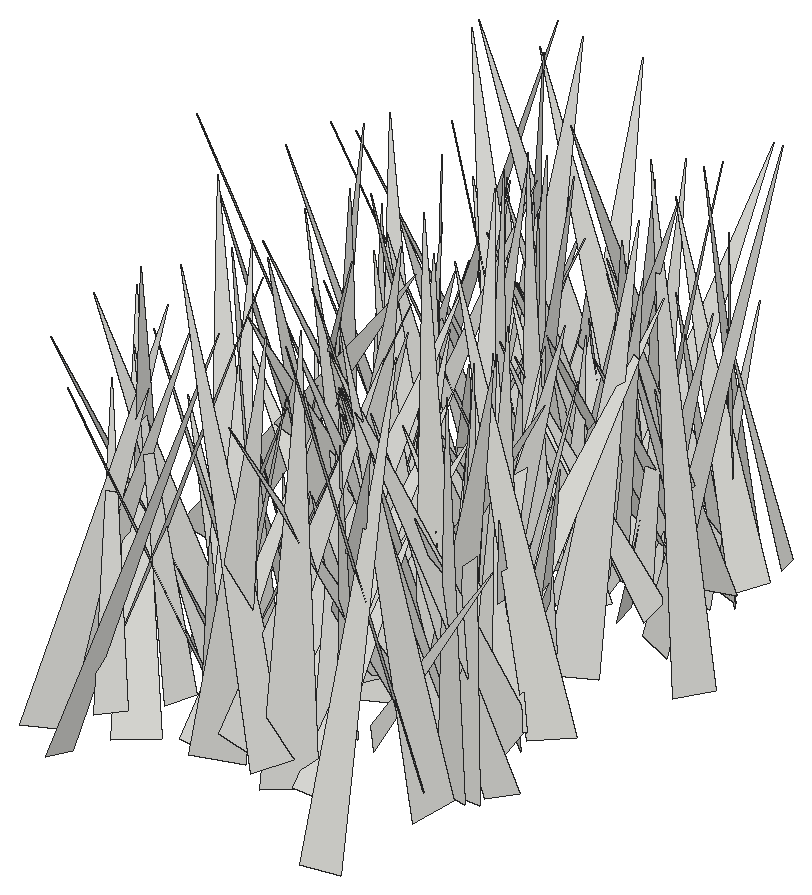
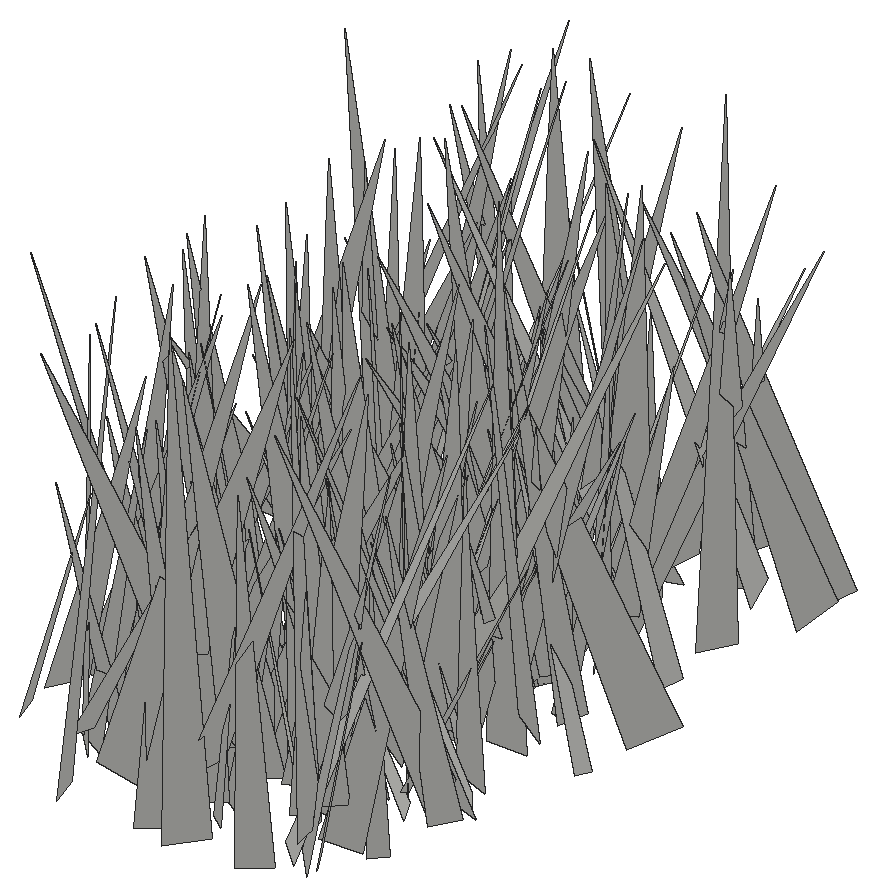
# SketchUp Ruby script. Lengths in inches.
U = 1.inch
M = Sketchup.active_model
def pt(a) = Geom::Point3d.new(a.map { |v| v * U })
def face(e, loops, mat)
  f = e.add_face(loops[0].map { |a| pt(a) })
  loops[1..].each { |l| e.add_face(l.map { |a| pt(a) }).erase! }
  f.material = f.back_material = mat if mat
  f
end
# faces: each face lists its corners as indices into pts; further lists are holes
def faces(e, pts, list, mat = nil) = list.each { |f| face(e, (f[0].is_a?(Array) ? f : [f]).map { |l| l.map { |i| pts[i] } }, mat) }
# xy, xz, yz: faces in a plane at the given z, y or x. An outline is a flat list of corners, or four numbers for a rectangle; further outlines are holes
def ring(l) = l.size == 4 ? [[l[0], l[1]], [l[2], l[1]], [l[2], l[3]], [l[0], l[3]]] : l.each_slice(2).to_a
def flat(e, list, mat, &to3) = list.each { |f| face(e, (f[0].is_a?(Array) ? f : [f]).map { |l| ring(l).map { |u, v| to3.(u, v) } }, mat) }
def xy(e, z, list, mat = nil) = flat(e, list, mat) { |x, y| [x, y, z] }
def xz(e, y, list, mat = nil) = flat(e, list, mat) { |x, z| [x, y, z] }
def yz(e, x, list, mat = nil) = flat(e, list, mat) { |y, z| [x, y, z] }
def lines(e, pts, list) = list.each { |a, b| e.add_line(pt(pts[a]), pt(pts[b])) }
# prism: a flat outline (further loops are holes) pulled along v
def prism(e, loops, v, mat = nil)
  f = face(e, loops, mat); d = Geom::Vector3d.new(v.map { |x| x * U })
  f.pushpull(f.normal.samedirection?(d) ? d.length : -d.length)
end
def box(e, o, s, mat = nil) = prism(e, [[o, [o[0] + s[0], o[1], o[2]], [o[0] + s[0], o[1] + s[1], o[2]], [o[0], o[1] + s[1], o[2]]]], [0, 0, s[2]], mat)
def at(x, y, z, deg = 0) = Geom::Transformation.translation(pt([x, y, z])) * Geom::Transformation.rotation(ORIGIN, Z_AXIS, deg.degrees)
def axes(o, x, y, z) = Geom::Transformation.new([*x, 0, *y, 0, *z, 0, *pt(o).to_a, 1])
def part(name) = M.definitions.add(name)
# library, detail: a bought-in or finely detailed component or shape, given as its bounding box
def library(name, o, s) = part(name).tap { |d| box(d.entities, o, s) }
def detail(e, o, s) = box(e.add_group.entities, o, s)
def put(e, d, t, mat = nil) = e.add_instance(d, t).tap { |i| i.material = mat if mat }
def group(e, t, mat = nil) = e.add_group.tap { |g| g.transformation = t; g.material = mat if mat }.entities
root = M.entities
c1 = part("fur_instance\#9")
p = [[0.8125,0,1.79],[0.67,-0.02,1.48],[0,-0.11,0],[0,0.11,0]]
faces(c1.entities,p,[[0,1,2,3]])
put(root,c1,axes([100.51,106.02,-27.1],[7.12647,2.20024,1.82821],[1.44023,-6.99989,2.8102],[-2.47167,2.26505,6.90872]))
put(root,c1,axes([101.21,101.27,-27.1],[3.25616,5.95918,2.11371],[6.15078,-3.5363,0.49462],[-1.46542,-1.60155,6.77272]))
put(root,c1,axes([104.27,100.93,-27.1],[-5.74525,-5.95088,0.61636],[-5.93253,5.55629,-1.65334],[-0.77329,1.58601,8.10478]))
put(root,c1,axes([100.38,88.77,-28.22],[6.0321,-2.57805,3.10449],[-3.62742,-5.91038,2.14001],[-1.76807,3.33038,6.20104]))
put(root,c1,axes([101.87,103.09,-28.22],[1.00537,5.49165,1.69021],[5.63183,-1.28199,0.81538],[-1.13911,-1.49133,5.52306]))
put(root,c1,axes([99.68,106.9375,-27.1],[3.13596,-3.23192,0.2957],[-3.22644,-3.06024,0.76944],[0.35051,0.74607,4.43707]))
put(root,c1,axes([99.99,94.38,-27.1],[7.80174,-0.94154,1.76979],[-0.49694,-7.7978,-1.95786],[-1.94209,-1.78708,7.61055]))
put(root,c1,axes([100.17,89.63,-28.22],[6.56769,-0.93589,1.93904],[-1.50422,-6.44796,1.98276],[-1.54048,2.30611,6.3308]))
put(root,c1,axes([103.04,89.9375,-28.22],[-5.19034,4.80556,0.45379],[4.78626,5.21014,-0.43029],[0.62529,0.00866,7.0603]))
put(root,c1,axes([104.52,106.3,-27.1],[-5.23491,-4.53939,0.15815],[-4.43832,5.06084,-1.65066],[-0.96564,1.34804,6.72946]))
put(root,c1,axes([103.82,94.04,-28.22],[-3.14306,-6.22127,0.26286],[-6.12359,3.03481,-1.39417],[-1.12913,0.859,6.8293]))
put(root,c1,axes([102.6,109.61,-28.22],[3.77255,3.78798,3.73229],[4.48771,-4.72284,0.25719],[-2.85294,-2.4201,5.33992]))
put(root,c1,axes([102.81,104.98,-28.22],[-3.84083,-1.16764,0.10273],[-1.10793,3.73134,0.98769],[0.38264,-0.91633,3.89099]))
put(root,c1,axes([102.65,89.2,-27.1],[-4.5808,2.50643,0.71678],[2.42315,4.62824,-0.69815],[0.96142,0.27723,5.1748]))
put(root,c1,axes([102.26,109.38,-28.22],[-3.18222,-1.83698,0.96818],[-1.93012,3.2701,-0.13938],[0.76583,0.60852,3.67173]))
put(root,c1,axes([103.26,109.46,-28.22],[-5.30348,-5.59312,0.1785],[-5.55783,5.29332,0.73008],[0.65218,-0.37354,7.67313]))
put(root,c1,axes([101.02,104.08,-28.22],[3.76049,3.04894,0.61025],[2.98388,-3.80785,0.6375],[-0.87456,0.11813,4.79905]))
put(root,c1,axes([103.05,99.85,-27.1],[-3.74984,-6.28849,1.24601],[-6.40364,3.74219,-0.38514],[0.30173,1.26879,7.3115]))
put(root,c1,axes([102.12,98.71,-28.22],[-1.40933,-4.17013,0.64925],[-4.20295,1.44894,0.18319],[0.38311,0.55526,4.39803]))
put(root,c1,axes([102.42,108.22,-28.22],[1.73584,-5.70606,0.92261],[-5.63591,-1.88469,-1.0526],[-1.28332,0.55882,5.87063]))
put(root,c1,axes([103.38,93.79,-27.1],[-6.6748,0.96554,1.83268],[1.43583,6.61336,1.7452],[1.49311,-2.0433,6.51456]))
put(root,c1,axes([99.69,100.75,-28.22],[5.19096,1.17327,0.15724],[1.14991,-4.82989,-1.92283],[0.28108,-1.90867,4.96239]))
put(root,c1,axes([103.83,92.53,-27.1],[-3.87501,-4.05549,0.17386],[-4.05477,3.85598,-0.42797],[-0.18982,0.42113,5.59281]))
put(root,c1,axes([103.15,102.8,-27.1],[-2.95923,6.17255,1.7602],[6.41346,2.92118,0.53848],[0.25723,-1.82266,6.82403]))
put(root,c1,axes([104.47,98.6,-27.1],[-4.30239,2.31555,0.00735],[2.25428,4.18495,1.12996],[-0.52922,-0.99839,4.75348]))
put(root,c1,axes([103.28,104.78,-27.1],[-2.87551,-4.98025,1.4124],[-5.17006,2.84441,-0.49611],[0.26119,1.47404,5.72934]))
put(root,c1,axes([103.24,94.57,-27.1],[-3.28307,2.60382,1.30489],[2.8552,3.26547,0.66758],[0.57484,-1.34832,4.13676]))
put(root,c1,axes([103.84,91.13,-27.1],[-5.54027,1.19429,0.93196],[1.15956,5.61711,-0.30487],[0.97482,0.10593,5.65933]))
put(root,c1,axes([104.51,97.04,-28.22],[-4.27144,-3.27285,0.83505],[-3.36103,3.98484,-1.57435],[-0.33515,1.75031,5.14569]))
put(root,c1,axes([104.72,106.42,-28.22],[-1.19348,5.65379,0.3473],[5.3271,0.99964,2.033],[-1.92561,-0.73875,5.40894]))
put(root,c1,axes([102.29,106.57,-27.1],[2.52877,4.50107,1.40807],[4.66336,-2.62485,0.01569],[-0.70386,-1.21962,5.16276]))
put(root,c1,axes([101.17,108.07,-28.22],[-0.15941,-4.26775,0.08772],[-3.87813,0.18147,1.78158],[1.78369,0.01316,3.88138]))
put(root,c1,axes([104.26,93.27,-27.1],[-3.06885,7.2619,1.47031],[7.40414,2.94663,0.90053],[-0.27521,-1.70206,7.83212]))
put(root,c1,axes([100.6,100.08,-27.1],[6.84395,0.46131,0.76105],[0.6015,-6.74756,-1.31919],[-0.65589,-1.3745,6.73144]))
put(root,c1,axes([103.05,109.02,-27.1],[1.88047,-2.78184,1.95652],[-3.20631,-2.19563,-0.04014],[-1.13412,1.59479,3.35756]))
put(root,c1,axes([98.13,99.47,-27.1],[4.31656,-7.06636,0.27005],[-6.24466,-3.6606,4.0303],[3.31821,2.3034,7.23345]))
put(root,c1,axes([105.06,106.08,-28.22],[-5.00695,6.61488,0.9269],[6.67749,4.92855,0.89773],[-0.16413,-1.27989,8.24744]))
put(root,c1,axes([104.67,94.05,-27.1],[-5.00716,-3.11226,0.75462],[-3.18598,4.98296,-0.58898],[0.32424,0.90067,5.86608]))
put(root,c1,axes([101.75,87.81,-28.22],[7.02888,1.27959,1.54515],[0.73768,-6.88381,2.34499],[-1.86566,2.099,6.7486]))
put(root,c1,axes([103.39,99.53,-27.1],[0.25291,3.93977,0.05992],[3.89833,-0.25892,0.57035],[-0.57304,-0.02262,3.90646]))
put(root,c1,axes([100.89,104.51,-28.22],[3.55811,5.92159,0.8478],[5.93377,-3.36884,-1.37307],[0.75783,-1.4247,6.77052]))
put(root,c1,axes([103.48,101.51,-28.22],[1.92833,-3.54748,0.58332],[-3.33012,-2.01195,-1.22706],[-1.35468,-0.10385,3.84674]))
put(root,c1,axes([101.02,91.1875,-27.1],[6.96857,2.87265,0.80723],[2.85827,-7.01507,0.2896],[-0.85676,-0.03815,7.53188]))
put(root,c1,axes([105.3,101.82,-27.1],[-6.81995,-3.62088,0.84533],[-3.65528,6.85252,-0.13797],[0.68141,0.51893,7.72033]))
put(root,c1,axes([103.89,97.78,-28.22],[-4.07522,2.66076,1.05763],[2.66001,4.19896,-0.31421],[1.05952,-0.30776,4.85678]))
put(root,c1,axes([102.33,109.73,-27.1],[7.07527,1.73735,2.55738],[2.12787,-7.36989,-0.88027],[-2.24293,-1.5114,7.23207]))
put(root,c1,axes([103.35,95.67,-28.22],[-4.27511,-3.26782,2.05551],[-3.38668,4.64678,0.34365],[1.85313,0.95347,5.37002]))
put(root,c1,axes([103.875,101.96,-28.22],[-3.24466,-1.65637,0.06319],[-1.44148,2.88818,1.68993],[0.81834,-1.47993,3.2273]))
put(root,c1,axes([102.73,104.83,-28.22],[5.50119,4.10651,2.99111],[4.73487,-5.74232,-0.82461],[-1.84151,-2.49711,6.81516]))
put(root,c1,axes([102.26,100.96,-28.22],[-1.23371,-7.71978,2.49826],[-7.92295,1.69122,1.31342],[1.75022,2.21429,7.70662]))
put(root,c1,axes([100.95,95.22,-28.22],[6.07626,0.90493,0.17774],[0.92213,-5.94508,-1.25588],[0.01299,-1.26833,6.01354]))
put(root,c1,axes([102.37,102.95,-27.1],[3.27913,1.40298,0.59687],[1.4938,-3.23974,-0.59158],[-0.30522,-0.78299,3.51725]))
put(root,c1,axes([104.22,107.05,-28.22],[-0.54447,5.56352,1.73211],[5.79599,0.33809,0.73596],[-0.59958,-1.78391,5.54144]))
put(root,c1,axes([103.5,98.86,-27.1],[2.79577,3.11606,1.7882],[3.42019,-3.00212,-0.11591],[-1.09992,-1.41467,4.18482]))
put(root,c1,axes([104.14,103.03,-28.22],[-6.0329,-5.73941,0.68236],[-5.34499,5.91535,2.49841],[2.19943,-1.36753,7.94322]))
put(root,c1,axes([103.9375,94.66,-27.1],[-4.03311,-0.04964,1.55556],[-0.10181,4.31995,-0.1261],[1.55302,0.15428,4.03144]))
put(root,c1,axes([104.72,100.72,-27.1],[-3.60372,1.36671,1.25031],[1.68423,3.55609,0.96723],[0.77106,-1.37995,3.73084]))
put(root,c1,axes([103.48,97.14,-28.22],[3.2467,-2.02133,0.75684],[-1.94033,-3.33216,-0.57574],[-0.94537,-0.10279,3.78092]))
put(root,c1,axes([106.92,108.78,-27.1],[-8.06825,0.70999,0.37952],[0.71569,8.07597,0.10667],[0.36866,-0.13964,8.09873]))
put(root,c1,axes([102.64,98.47,-27.1],[0.8957,-3.44027,0.95903],[-3.38159,-0.49886,1.36875],[1.14894,1.21373,3.28089]))
put(root,c1,axes([102.89,108.24,-27.1],[3.51068,-4.45404,1.06123],[-4.56743,-3.50052,0.41776],[-0.32136,1.09429,5.65587]))
put(root,c1,axes([103.93,95.55,-28.22],[3.63401,0.67625,1.41653],[0.37628,-3.84346,0.86953],[-1.5239,0.6636,3.59267]))
put(root,c1,axes([106.34,101.19,-27.1],[-4.80301,-2.64529,0.12183],[-2.62964,4.73476,-0.865],[-0.31202,0.81591,5.41463]))
put(root,c1,axes([105.0625,100.73,-28.22],[-6.05732,0.47074,1.68041],[-0.07648,5.99257,-1.95441],[1.74342,1.89841,5.75265]))
put(root,c1,axes([102.79,99.89,-27.1],[4.10289,-2.86128,0.97197],[-3.01034,-4.01302,0.89377],[-0.2636,1.29386,4.92156]))
put(root,c1,axes([105.2,91.62,-27.1],[-2.95766,6.66869,1.17233],[6.76114,2.97762,0.11972],[0.36439,-1.12067,7.29416]))
put(root,c1,axes([103.08,106.51,-27.1],[5.00649,-0.69371,1.01239],[-0.92226,-4.93206,1.18126],[-0.80969,1.32843,4.91435]))
put(root,c1,axes([104.04,101.21,-28.22],[3.31226,-1.52366,0.97308],[-1.49474,-3.45052,-0.31491],[-1.01694,0.10903,3.63228]))
put(root,c1,axes([106.28,92.62,-27.1],[-7.03444,-1.19576,1.59787],[-1.52444,6.99776,-1.47438],[1.28808,1.75153,6.98136]))
put(root,c1,axes([104.12,105.61,-27.1],[2.60004,3.22909,0.64132],[3.22546,-2.66223,0.32783],[-0.65933,-0.2899,4.13277]))
put(root,c1,axes([102.19,105.55,-28.22],[5.45999,3.37552,0.2587],[3.37248,-5.38033,-0.97518],[0.29572,-0.96459,6.34466]))
put(root,c1,axes([107.52,95.59,-27.1],[-7.36083,-0.13148,0.37404],[-0.23398,7.05478,-2.12469],[0.32007,2.13349,7.04874]))
put(root,c1,axes([104.99,97.65,-27.1],[0.47812,-7.3143,1.47747],[-7.45136,-0.54714,-0.29732],[-0.39895,1.45332,7.32388]))
put(root,c1,axes([105.33,101.18,-28.22],[3.75973,-6.87339,0.18092],[-6.4988,-3.61971,-2.46477],[-2.2454,-1.03249,7.43666]))
put(root,c1,axes([105.29,106.36,-27.1],[-1.61358,3.38665,0.61033],[3.4322,1.63258,0.01498],[0.24881,-0.55751,3.75138]))
put(root,c1,axes([103.53,110.6875,-28.22],[2.32363,-4.81619,0.47979],[-4.81966,-2.25368,0.71896],[0.44354,0.74187,5.29887]))
put(root,c1,axes([104.67,102.02,-27.1],[4.30224,-3.16543,2.15858],[-3.43037,-4.62804,0.05027],[-1.70646,1.32286,5.34104]))
put(root,c1,axes([103.14,108.71,-28.22],[3.99613,2.0991,0.80323],[2.24013,-3.58697,-1.77087],[0.18236,-1.93595,4.15203]))
put(root,c1,axes([106.1875,99.52,-28.22],[-1.23354,6.12021,2.2306],[6.48252,0.93032,1.03231],[-0.63996,-2.37312,6.15735]))
put(root,c1,axes([104.78,105.72,-27.1],[-2.78975,7.45432,2.27613],[7.61508,3.12201,-0.8911],[1.66081,-1.79348,7.90921]))
put(root,c1,axes([104.54,91.85,-28.22],[3.43508,-2.31671,0.74566],[-2.27877,-3.51457,-0.42176],[-0.85461,0.05948,4.12177]))
put(root,c1,axes([106.88,99.83,-27.1],[-1.92431,3.57441,0.40694],[3.46774,1.72017,1.28872],[-0.95749,-0.95373,3.84949]))
put(root,c1,axes([104.73,90.71,-28.22],[-0.26942,5.43204,0.24352],[5.36362,0.30555,-0.88154],[0.89325,-0.19629,5.36679]))
put(root,c1,axes([105.9375,95.84,-27.1],[-2.69846,2.82224,0.09608],[2.72603,2.63813,-0.93001],[0.73688,0.57546,3.79233]))
put(root,c1,axes([104.32,94.65,-28.22],[1.94389,-4.04886,0.80465],[-4.08173,-1.75236,1.04312],[0.61659,1.16421,4.36851]))
put(root,c1,axes([106.88,101.97,-28.22],[4.68158,-4.31782,3.21331],[-4.18207,-5.59908,-1.43065],[-3.3881,0.94493,6.20597]))
put(root,c1,axes([105.06,91.43,-28.22],[-3.61899,-3.55384,3.43713],[-4.24844,4.41399,0.09065],[2.52873,2.32973,5.07136]))
put(root,c1,axes([108.56,89.64,-27.1],[-7.87651,1.28049,0.44694],[1.23259,7.85729,-0.78901],[0.56579,0.70864,7.94081]))
put(root,c1,axes([104.18,101.01,-28.22],[1.15805,-3.96128,0.43832],[-3.70743,-0.90324,1.63219],[1.46246,0.84697,3.79062]))
put(root,c1,axes([106.32,108.28,-28.22],[-1.9321,-3.03286,0.9193],[-3.13143,1.99261,-0.00754],[0.48737,0.77951,3.596]))
put(root,c1,axes([106.08,101.64,-28.22],[-6.74927,1.80081,2.69667],[1.18797,7.16726,-1.81295],[3.01723,1.2063,6.74602]))
put(root,c1,axes([105.99,109.3,-28.22],[-2.25784,-3.06403,1.232],[-3.11024,2.47464,0.4545],[1.1102,0.70132,3.77883]))
put(root,c1,axes([104.39,98.34,-28.22],[5.49312,-5.94068,1.74056],[-6.16398,-5.4638,0.80479],[-0.57141,1.8305,8.05098]))
put(root,c1,axes([106.73,106.67,-28.22],[-3.53884,7.24303,1.02774],[7.25201,3.62348,-0.56563],[0.96238,-0.67082,8.04145]))
put(root,c1,axes([107.43,103.75,-27.1],[1.37607,4.21587,0.41156],[3.82506,-1.42264,1.78368],[-1.81985,0.19763,4.06025]))
put(root,c1,axes([107.39,106.15,-28.22],[-0.21744,-4.53269,0.61909],[-4.46943,0.07824,-0.99696],[-0.9761,0.65149,4.42703]))
put(root,c1,axes([108.73,107.24,-27.1],[-1.67937,-5.43767,0.87836],[-5.25266,1.30456,-1.96667],[-1.65811,1.37475,5.34049]))
put(root,c1,axes([104.1,92.5,-28.22],[7.40183,3.33475,0.3809],[3.31775,-7.40888,0.39208],[-0.5081,0.20159,8.10888]))
put(root,c1,axes([105.26,95.05,-27.1],[-1.51128,6.4389,0.97646],[6.11666,1.74753,-2.05657],[2.23592,-0.42848,6.28601]))
put(root,c1,axes([106.66,102.9,-28.22],[4.08531,-1.79648,1.28746],[-1.24322,-4.1049,-1.78292],[-1.82737,-1.22355,4.09124]))
put(root,c1,axes([109.89,107.04,-27.1],[-2.9065,7.574,1.65107],[7.44857,2.24028,2.83534],[-2.14716,-2.4809,7.60092]))
put(root,c1,axes([105.74,90.5,-28.22],[-3.12669,6.25889,3.83958],[6.87271,3.96367,-0.86451],[2.58493,-2.9678,6.9428]))
put(root,c1,axes([108.35,106.79,-27.1],[-6.30832,-1.1114,1.05664],[-1.00602,6.37534,0.69964],[1.15742,-0.51611,6.36715]))
put(root,c1,axes([106.97,107.16,-27.1],[3.89618,-1.88557,1.1779],[-1.51971,-3.99347,-1.36592],[-1.62275,-0.78732,4.1073]))
put(root,c1,axes([108.54,92.37,-27.1],[-4.64664,1.60589,0.29185],[1.45378,4.47236,-1.46283],[0.74202,1.29401,4.69365]))
put(root,c1,axes([107.36,96.37,-28.22],[-4.4871,3.83069,1.41429],[3.5666,4.69982,-1.41404],[1.98841,0.2144,5.72789]))
put(root,c1,axes([107.625,105.37,-27.1],[-1.75963,-5.21212,1.71135],[-5.46295,1.82898,-0.04671],[0.50104,1.63703,5.50093]))
put(root,c1,axes([107.24,95.7,-27.1],[2.57242,-3.23839,0.522],[-3.12857,-2.6216,-0.84629],[-0.98573,-0.13048,4.04824]))
put(root,c1,axes([106.1,101.11,-27.1],[3.40491,-1.73217,0.1961],[-1.74293,-3.39081,0.31125],[-0.03288,0.3664,3.80749]))
put(root,c1,axes([108.74,102.625,-27.1],[-0.19761,-4.29399,0.26182],[-4.09062,0.10641,-1.34218],[-1.33181,0.31028,4.08362]))
put(root,c1,axes([105.92,110.75,-28.22],[6.83248,-2.68093,1.04491],[-2.55055,-6.88917,-0.99801],[-1.33189,-0.56029,7.27146]))
put(root,c1,axes([106.04,94.7,-28.22],[-1.05033,5.0969,0.69056],[4.61293,1.24522,-2.17458],[2.27512,-0.17172,4.72788]))
put(root,c1,axes([106.82,92.95,-28.22],[-2.16647,5.60636,0.16983],[5.26617,2.09582,-2.00715],[1.93067,0.57445,5.66535]))
put(root,c1,axes([106.44,103.96,-28.22],[7.78387,0.2727,2.09642],[0.3333,-8.05673,-0.18953],[-2.08764,-0.26953,7.78634]))
put(root,c1,axes([108.61,110.46,-27.1],[-0.93689,-7.58778,0.99671],[-7.63501,0.85799,-0.64504],[-0.52389,1.06539,7.61814]))
put(root,c1,axes([110.06,103.4,-27.1],[-3.00277,4.1066,0.06153],[3.92812,2.84936,1.52829],[-1.19912,-0.94951,4.85234]))
put(root,c1,axes([107.27,103.14,-28.22],[7.52534,-2.11015,2.94691],[-2.32099,-8.02168,0.183],[-2.78389,0.98374,7.81345]))
put(root,c1,axes([108.97,98.64,-28.22],[5.53383,-2.65462,5.00816],[-4.23304,-6.59023,1.18414],[-3.76962,3.5034,6.0223]))
put(root,c1,axes([107.43,103.99,-28.22],[-6.42267,-1.42598,3.31634],[-1.29179,7.22813,0.60623],[3.37087,0.05298,6.55107]))
put(root,c1,axes([107.8,105.02,-27.1],[0.95056,-3.70171,1.6828],[-4.06505,-0.90725,0.30052],[-0.09921,1.70654,3.80998]))
put(root,c1,axes([110.11,98.27,-27.1],[-7.67594,0.43258,1.18162],[-0.05572,7.18028,-2.99063],[1.25708,2.9597,7.0826]))
put(root,c1,axes([109.02,97.25,-27.1],[-5.87389,-5.06073,1.31002],[-4.91563,6.01764,1.20596],[1.77871,-0.08191,7.65893]))
put(root,c1,axes([108.75,97.4,-27.1],[-6.83559,-3.49227,1.59422],[-2.83471,6.78714,2.71329],[2.5888,-1.7893,7.18049]))
put(root,c1,axes([107.1,110.64,-28.22],[5.27759,-3.33069,0.22963],[-3.2336,-5.20637,-1.19863],[-0.83073,-0.89406,6.12452]))
put(root,c1,axes([109.5,107.26,-27.1],[-1.38983,-5.84462,0.0201],[-5.82782,1.38425,-0.46046],[-0.44334,0.12603,5.98992]))
put(root,c1,axes([106.98,89.98,-27.1],[0.16958,6.97336,1.46095],[6.91324,0.19239,-1.72074],[1.72314,-1.45812,6.75984]))
put(root,c1,axes([109.55,106.38,-28.22],[0.68594,6.83231,0.78357],[6.74689,-0.82108,1.2531],[-1.33188,-0.64057,6.75135]))
put(root,c1,axes([108.59,90.4375,-28.22],[4.92232,-5.34816,3.43981],[-5.97476,-5.37881,0.1869],[-2.17654,2.67018,7.26616]))
put(root,c1,axes([109.23,95.3,-27.1],[-5.37416,-4.85351,0.14678],[-4.51514,5.07548,2.5125],[1.7865,-1.77274,6.79157]))
put(root,c1,axes([109.8125,104.55,-27.1],[-4.7933,-0.97536,0.74224],[-0.77682,4.73507,1.20565],[0.94805,-1.05153,4.74061]))
put(root,c1,axes([109.78,96.2,-27.1],[-0.81741,7.52572,2.31704],[7.8363,0.54876,0.98214],[-0.77303,-2.39493,7.506]))
put(root,c1,axes([107.38,105.2,-27.1],[4.01593,3.70117,1.52807],[3.99587,-3.8439,-1.19115],[-0.25835,-1.92018,5.32987]))
put(root,c1,axes([110.3,100.37,-27.1],[0.70044,7.59304,1.85976],[7.56257,-1.13109,1.76971],[-1.98005,-1.63401,7.41708]))
put(root,c1,axes([110.18,96.23,-27.1],[-4.46035,-2.40279,1.6408],[-2.85913,4.17643,-1.65628],[0.53948,2.26814,4.788]))
put(root,c1,axes([106.26,98.57,-27.1],[4.90095,-2.69617,0.00541],[-2.57457,-4.67657,1.67032],[0.80058,1.46597,5.33842]))
put(root,c1,axes([106.6,106.22,-28.22],[7.07738,-3.29601,0.99897],[-3.4049,-7.03943,0.89669],[-0.51794,1.23844,7.75557]))
put(root,c1,axes([110.91,109.22,-27.1],[-4.62797,0.36048,0.06702],[0.36662,4.56134,0.78248],[0.00509,-0.78533,4.57556]))
put(root,c1,axes([109.2,102.86,-27.1],[-3.77654,1.99621,0.89861],[1.50689,3.67022,-1.82025],[1.58796,1.26459,3.86442]))
put(root,c1,axes([108.96,92.82,-27.1],[-1.48378,-4.80354,1.85374],[-5.06695,1.70492,0.36217],[0.91449,1.65264,5.01442]))
put(root,c1,axes([109.36,99.04,-27.1],[-0.62067,4.74172,0.56344],[4.77083,0.63973,-0.12835],[0.20124,-0.5417,4.78044]))
put(root,c1,axes([107.07,108.68,-28.22],[1.43301,-8.2393,0.15598],[-8.02359,-1.35888,1.93375],[1.87948,0.48092,8.13635]))
put(root,c1,axes([108,100.8,-27.1],[-1.7832,4.7887,2.83203],[5.02838,2.65983,-1.33139],[2.38064,-2.03113,4.93345]))
put(root,c1,axes([111.05,98.07,-27.1],[-4.33776,1.46199,0.55548],[1.55819,4.18055,1.16497],[0.13425,-1.28363,4.42678]))
put(root,c1,axes([108.36,107.98,-28.22],[1.50872,-5.62418,0.24688],[-5.60162,-1.47433,0.64555],[0.56049,0.40439,5.78713]))
put(root,c1,axes([106.74,95.11,-27.1],[-0.05965,-7.49908,0.31223],[-6.76708,0.1888,3.24163],[3.24657,0.25574,6.76251]))
put(root,c1,axes([111.43,94.31,-27.1],[-5.40823,0.65228,0.52882],[0.69912,5.40686,0.48075],[0.46513,-0.5426,5.42617]))
put(root,c1,axes([109.23,90.55,-28.22],[-1.55041,4.4226,0.08121],[4.26043,1.51619,-1.23272],[1.18941,0.33394,4.52145]))
put(root,c1,axes([111.12,94.78,-27.1],[-1.48365,-5.76059,1.44193],[-5.8771,1.21156,-1.20691],[-0.85046,1.67706,5.82486]))
put(root,c1,axes([108.73,106.28,-27.1],[-1.75958,6.89289,0.89816],[6.66639,1.93582,-1.79628],[1.96924,-0.39424,6.88342]))
put(root,c1,axes([111.65,104.34,-27.1],[-4.90231,-0.23018,0.15933],[-0.18525,4.76264,1.18065],[0.20988,-1.17272,4.76358]))
put(root,c1,axes([109.88,96.73,-28.22],[3.30572,4.13092,2.03155],[4.38871,-3.58299,0.14433],[-1.38957,-1.489,5.28881]))
put(root,c1,axes([109.34,104.12,-27.1],[4.20018,-2.603,1.54886],[-2.85846,-4.28223,0.55487],[-1.0019,1.30501,4.91012]))
put(root,c1,axes([109.79,105.18,-28.22],[6.4621,3.38539,1.99868],[3.00841,-6.73382,1.67909],[-2.53082,0.63956,7.09931]))
put(root,c1,axes([111.08,107.27,-27.1],[-0.25255,-4.7231,0.0991],[-4.68784,0.23828,-0.59045],[-0.58449,0.12972,4.69284]))
put(root,c1,axes([110.43,110.61,-28.22],[-6.30807,-3.21691,2.7037],[-2.95993,6.86307,1.25992],[2.98285,0.00727,6.96799]))
put(root,c1,axes([109.55,106.82,-27.1],[4.23339,-1.74729,1.15695],[-1.93705,-4.25778,0.65751],[-0.79963,1.0637,4.53236]))
put(root,c1,axes([109.02,105.33,-27.1],[1.26894,-6.32164,1.3833],[-6.3592,-0.957,1.46001],[1.19887,1.6149,6.28026]))
put(root,c1,axes([110.53,104.99,-27.1],[0.04059,4.23783,1.33242],[4.44047,0.00019,-0.13586],[0.12965,-1.33303,4.23585]))
put(root,c1,axes([111.52,108.03,-28.22],[-2.15143,-4.58063,1.63472],[-4.86135,2.07952,-0.57094],[0.14745,1.72526,5.02841]))
put(root,c1,axes([112.61,91.73,-27.1],[-5.20648,-5.71637,1.32602],[-5.85189,5.18966,-0.6046],[0.43665,1.3904,7.70836]))
put(root,c1,axes([110.04,98.23,-27.1],[-2.9172,5.75801,0.16061],[5.28877,2.74872,-2.48273],[2.2824,0.99014,5.95825]))
put(root,c1,axes([112.99,107.3,-27.1],[-5.78073,2.46703,0.60773],[2.49572,5.79658,0.20851],[0.47643,-0.43109,6.28168]))
put(root,c1,axes([110.64,97.96,-27.1],[3.75494,-4.9741,2.2471],[-5.32599,-3.93562,0.18806],[-1.1937,1.91308,6.22943]))
put(root,c1,axes([112.44,106.57,-27.1],[-0.64276,-5.9949,1.38637],[-6.03632,0.34404,-1.31091],[-1.1932,1.48889,5.88502]))
put(root,c1,axes([110.95,101.19,-28.22],[-4.71435,5.59524,2.23508],[5.56124,5.13291,-1.11952],[2.31839,-0.93486,7.23039]))
put(root,c1,axes([111.55,96.12,-28.22],[2.78013,5.13783,0.11647],[4.85085,-2.66723,1.86951],[-1.69707,0.79284,5.53456]))
put(root,c1,axes([110.66,107.3,-27.1],[4.01864,-1.00258,0.99057],[-0.63294,-3.95809,-1.43832],[-1.25928,-1.21004,3.88405]))
put(root,c1,axes([111.11,107.1875,-28.22],[1.25627,4.75609,0.70963],[4.78282,-1.31187,0.32531],[-0.49861,-0.60066,4.90844]))
put(root,c1,axes([112.89,92.07,-28.22],[-8.03417,0.61584,1.78735],[0.70083,8.21761,0.3188],[1.75577,-0.4621,8.05143]))
put(root,c1,axes([112.03,106.09,-27.1],[-5.14482,-3.13912,1.24988],[-3.04737,5.29445,0.7535],[1.4594,-0.01101,5.97959]))
put(root,c1,axes([112.84,95.79,-27.1],[-0.8171,5.77252,0.59098],[5.63961,0.64951,1.4532],[-1.36602,-0.77139,5.64605]))
put(root,c1,axes([113.92,94.14,-28.22],[-0.7555,-5.85213,2.53673],[-5.87032,-0.36099,-2.58111],[-2.49433,2.62211,5.30623]))
put(root,c1,axes([109.97,100.68,-27.1],[4.41728,-0.60705,0.29796],[-0.51929,-4.30631,-1.07505],[-0.43316,-1.02804,4.32726]))
put(root,c1,axes([113.37,95.49,-27.1],[-7.55604,-1.18176,1.01335],[-0.88861,7.39753,2.00103],[1.27821,-1.84315,7.38147]))
put(root,c1,axes([112.47,87.11,-28.22],[0.70826,8.01559,0.32411],[7.89046,-0.75477,1.42384],[-1.44754,-0.19233,7.91985]))
put(root,c1,axes([110.53,98.92,-28.22],[3.79566,-1.87078,0.73995],[-1.92959,-3.83243,0.2087],[-0.56925,0.51676,4.2265]))
put(root,c1,axes([111.73,96.84,-27.1],[1.96703,-4.29578,0.10046],[-4.18734,-1.94112,-1.01553],[-0.96439,-0.33368,4.61429]))
put(root,c1,axes([111.04,98.11,-27.1],[2.15592,-3.18911,0.31319],[-3.19535,-2.16794,-0.07942],[-0.24138,0.21478,3.84865]))
put(root,c1,axes([111.625,108.16,-28.22],[4.37424,4.04681,2.79179],[4.54542,-4.75288,-0.23239],[-1.87347,-2.08284,5.95454]))
put(root,c1,axes([114.12,96.27,-27.1],[-2.60972,7.0339,1.93347],[7.14895,2.0575,2.16424],[-1.45142,-2.51309,7.18348]))
put(root,c1,axes([112.33,96.9,-28.22],[-2.70575,-2.79772,1.42447],[-3.05403,2.78134,-0.3384],[0.7275,1.27058,3.87735]))
put(root,c1,axes([112.97,109.15,-27.1],[-3.79015,-1.11399,0.60809],[-1.15598,3.82064,-0.20588],[0.52388,0.37109,3.9451]))
put(root,c1,axes([114.53,102.67,-28.22],[-8.1921,1.36867,0.61461],[1.20152,8.02801,-1.8625],[0.89853,1.74336,8.09413]))
put(root,c1,axes([109.84,92.91,-27.1],[3.27011,3.05252,0.13659],[2.8317,-2.95233,-1.81533],[1.14804,-1.41282,4.08853]))
put(root,c1,axes([112.74,93.13,-28.22],[1.52535,6.05061,2.3847],[6.37233,-1.8801,0.69429],[-1.30004,-2.1163,6.20117]))
put(root,c1,axes([113.16,93.26,-28.22],[1.52535,6.57132,1.88983],[6.63248,-1.89273,1.22809],[-1.66251,-1.52175,6.63331]))
put(root,c1,axes([110.2,95.9375,-27.1],[1.15039,-7.47242,1.55869],[-7.41634,-0.72104,2.01691],[1.80677,1.79806,7.28646]))
put(root,c1,axes([111.76,104.24,-28.22],[3.85814,7.37241,1.12129],[7.37277,-3.96052,0.67189],[-1.11889,-0.67587,8.29374]))
